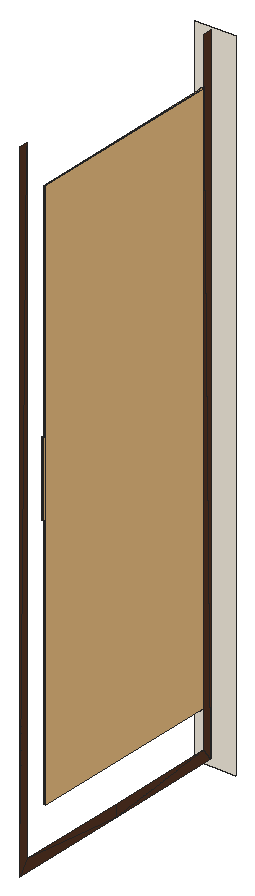
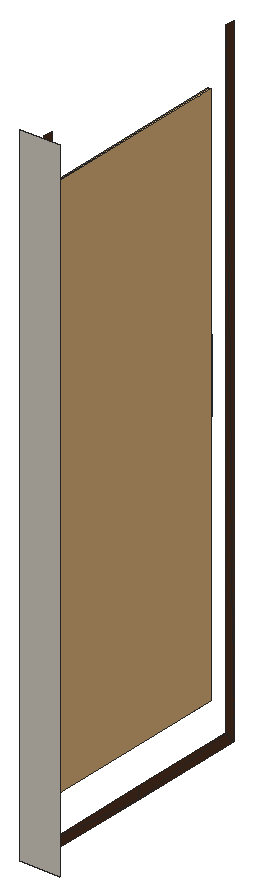
# SketchUp Ruby script. Lengths in inches.
U = 1.inch
M = Sketchup.active_model
def pt(a) = Geom::Point3d.new(a.map { |v| v * U })
def face(e, loops, mat)
  f = e.add_face(loops[0].map { |a| pt(a) })
  loops[1..].each { |l| e.add_face(l.map { |a| pt(a) }).erase! }
  f.material = f.back_material = mat if mat
  f
end
# faces: each face lists its corners as indices into pts; further lists are holes
def faces(e, pts, list, mat = nil) = list.each { |f| face(e, (f[0].is_a?(Array) ? f : [f]).map { |l| l.map { |i| pts[i] } }, mat) }
# xy, xz, yz: faces in a plane at the given z, y or x. An outline is a flat list of corners, or four numbers for a rectangle; further outlines are holes
def ring(l) = l.size == 4 ? [[l[0], l[1]], [l[2], l[1]], [l[2], l[3]], [l[0], l[3]]] : l.each_slice(2).to_a
def flat(e, list, mat, &to3) = list.each { |f| face(e, (f[0].is_a?(Array) ? f : [f]).map { |l| ring(l).map { |u, v| to3.(u, v) } }, mat) }
def xy(e, z, list, mat = nil) = flat(e, list, mat) { |x, y| [x, y, z] }
def xz(e, y, list, mat = nil) = flat(e, list, mat) { |x, z| [x, y, z] }
def yz(e, x, list, mat = nil) = flat(e, list, mat) { |y, z| [x, y, z] }
def lines(e, pts, list) = list.each { |a, b| e.add_line(pt(pts[a]), pt(pts[b])) }
# prism: a flat outline (further loops are holes) pulled along v
def prism(e, loops, v, mat = nil)
  f = face(e, loops, mat); d = Geom::Vector3d.new(v.map { |x| x * U })
  f.pushpull(f.normal.samedirection?(d) ? d.length : -d.length)
end
def box(e, o, s, mat = nil) = prism(e, [[o, [o[0] + s[0], o[1], o[2]], [o[0] + s[0], o[1] + s[1], o[2]], [o[0], o[1] + s[1], o[2]]]], [0, 0, s[2]], mat)
def at(x, y, z, deg = 0) = Geom::Transformation.translation(pt([x, y, z])) * Geom::Transformation.rotation(ORIGIN, Z_AXIS, deg.degrees)
def axes(o, x, y, z) = Geom::Transformation.new([*x, 0, *y, 0, *z, 0, *pt(o).to_a, 1])
def part(name) = M.definitions.add(name)
# library, detail: a bought-in or finely detailed component or shape, given as its bounding box
def library(name, o, s) = part(name).tap { |d| box(d.entities, o, s) }
def detail(e, o, s) = box(e.add_group.entities, o, s)
def put(e, d, t, mat = nil) = e.add_instance(d, t).tap { |i| i.material = mat if mat }
def group(e, t, mat = nil) = e.add_group.tap { |g| g.transformation = t; g.material = mat if mat }.entities
root = M.entities
M.materials.add("Material \#0").color = [86, 53, 35]
M.materials.add("Material \#1").color = [140, 140, 140]
M.materials.add("[0030_OldLace]").color = [253, 245, 230]
c1 = library("3DGeom~3_Defintion",[-83.33,-500,-350],[620.1,1000,533.33])
c2 = library("3DGeom~6_Defintion",[-5.59,-471.8,-48.03],[468.87,1000,73.72])
c3 = part("3DGeom~21_Defintion")
xy(c3.entities,73.08,[[-976.3,-241.71,23.7,-241.71,-976.3,-223.46],[23.7,-241.71,5.45,-223.46,-976.3,-223.46],[23.7,-241.71,23.7,0,5.45,-223.46],[5.45,-223.46,23.7,0,5.45,0],[23.7,0,23.7,241.71,5.45,223.46],
  [5.45,0,23.7,0,5.45,223.46],[-976.3,223.46,23.7,241.71,-976.3,241.71],[-976.3,223.46,5.45,223.46,23.7,241.71]],"Material \#0")
c4 = part("3DGeom~8_Defintion")
xz(c4.entities,-471.94,[[458.125,-17.29,459.53,-16.11,457.73,-17.15],[458.125,-17.29,458.54,-17.29,459.53,-16.11],[458.54,-17.29,458.93,-17.15,459.53,-16.11],[457.73,-17.15,459.53,-16.11,457.42,-16.88],[458.93,-17.15,459.25,-16.88,459.53,-16.11],
  [457.42,-16.88,459.53,-16.11,457.21,-16.52],[459.25,-16.88,459.46,-16.52,459.53,-16.11],[457.21,-16.52,459.53,-16.11,457.14,-16.11],[457.14,-16.11,459.53,-16.11,457.21,-15.7],[459.53,-16.11,457.42,-15.34,457.21,-15.7],
  [459.53,-16.11,457.73,-15.07,457.42,-15.34],[459.53,-16.11,458.125,-14.93,457.73,-15.07],[459.53,-16.11,458.54,-14.93,458.125,-14.93],[459.53,-16.11,458.93,-15.07,458.54,-14.93],[459.53,-16.11,459.25,-15.34,458.93,-15.07],
  [459.53,-16.11,459.46,-15.7,459.25,-15.34]],"Material \#1")
xz(c4.entities,-416.39,[[458.125,-17.29,457.73,-17.15,459.53,-16.11],[458.125,-17.29,459.53,-16.11,458.54,-17.29],[458.54,-17.29,459.53,-16.11,458.93,-17.15],[457.73,-17.15,457.42,-16.88,459.53,-16.11],[458.93,-17.15,459.53,-16.11,459.25,-16.88],
  [457.42,-16.88,457.21,-16.52,459.53,-16.11],[459.25,-16.88,459.53,-16.11,459.46,-16.52],[457.21,-16.52,457.14,-16.11,459.53,-16.11],[457.14,-16.11,457.21,-15.7,459.53,-16.11],[459.53,-16.11,457.21,-15.7,457.42,-15.34],
  [459.53,-16.11,457.42,-15.34,457.73,-15.07],[459.53,-16.11,457.73,-15.07,458.125,-14.93],[459.53,-16.11,458.125,-14.93,458.54,-14.93],[459.53,-16.11,458.54,-14.93,458.93,-15.07],[459.53,-16.11,458.93,-15.07,459.25,-15.34],
  [459.53,-16.11,459.25,-15.34,459.46,-15.7]],"Material \#1")
xz(c4.entities,-27.5,[[458.125,-17.29,459.53,-16.11,457.73,-17.15],[458.125,-17.29,458.54,-17.29,459.53,-16.11],[458.54,-17.29,458.93,-17.15,459.53,-16.11],[457.73,-17.15,459.53,-16.11,457.42,-16.88],[458.93,-17.15,459.25,-16.88,459.53,-16.11],
  [457.42,-16.88,459.53,-16.11,457.21,-16.52],[459.25,-16.88,459.46,-16.52,459.53,-16.11],[457.21,-16.52,459.53,-16.11,457.14,-16.11],[457.14,-16.11,459.53,-16.11,457.21,-15.7],[459.53,-16.11,457.42,-15.34,457.21,-15.7],
  [459.53,-16.11,457.73,-15.07,457.42,-15.34],[459.53,-16.11,458.125,-14.93,457.73,-15.07],[459.53,-16.11,458.54,-14.93,458.125,-14.93],[459.53,-16.11,458.93,-15.07,458.54,-14.93],[459.53,-16.11,459.25,-15.34,458.93,-15.07],
  [459.53,-16.11,459.46,-15.7,459.25,-15.34]],"Material \#1")
xz(c4.entities,28.06,[[458.125,-17.29,457.73,-17.15,459.53,-16.11],[458.125,-17.29,459.53,-16.11,458.54,-17.29],[458.54,-17.29,459.53,-16.11,458.93,-17.15],[457.73,-17.15,457.42,-16.88,459.53,-16.11],[458.93,-17.15,459.53,-16.11,459.25,-16.88],
  [457.42,-16.88,457.21,-16.52,459.53,-16.11],[459.25,-16.88,459.53,-16.11,459.46,-16.52],[457.21,-16.52,457.14,-16.11,459.53,-16.11],[457.14,-16.11,457.21,-15.7,459.53,-16.11],[459.53,-16.11,457.21,-15.7,457.42,-15.34],
  [459.53,-16.11,457.42,-15.34,457.73,-15.07],[459.53,-16.11,457.73,-15.07,458.125,-14.93],[459.53,-16.11,458.125,-14.93,458.54,-14.93],[459.53,-16.11,458.54,-14.93,458.93,-15.07],[459.53,-16.11,458.93,-15.07,459.25,-15.34],
  [459.53,-16.11,459.25,-15.34,459.46,-15.7]],"Material \#1")
xz(c4.entities,472.5,[[458.125,-17.29,459.53,-16.11,457.73,-17.15],[458.125,-17.29,458.54,-17.29,459.53,-16.11],[458.54,-17.29,458.93,-17.15,459.53,-16.11],[457.73,-17.15,459.53,-16.11,457.42,-16.88],[458.93,-17.15,459.25,-16.88,459.53,-16.11],
  [457.42,-16.88,459.53,-16.11,457.21,-16.52],[459.25,-16.88,459.46,-16.52,459.53,-16.11],[457.21,-16.52,459.53,-16.11,457.14,-16.11],[457.14,-16.11,459.53,-16.11,457.21,-15.7],[459.53,-16.11,457.42,-15.34,457.21,-15.7],
  [459.53,-16.11,457.73,-15.07,457.42,-15.34],[459.53,-16.11,458.125,-14.93,457.73,-15.07],[459.53,-16.11,458.54,-14.93,458.125,-14.93],[459.53,-16.11,458.93,-15.07,458.54,-14.93],[459.53,-16.11,459.25,-15.34,458.93,-15.07],
  [459.53,-16.11,459.46,-15.7,459.25,-15.34]],"Material \#1")
xz(c4.entities,528.06,[[458.125,-17.29,457.73,-17.15,459.53,-16.11],[458.125,-17.29,459.53,-16.11,458.54,-17.29],[458.54,-17.29,459.53,-16.11,458.93,-17.15],[457.73,-17.15,457.42,-16.88,459.53,-16.11],[458.93,-17.15,459.53,-16.11,459.25,-16.88],
  [457.42,-16.88,457.21,-16.52,459.53,-16.11],[459.25,-16.88,459.53,-16.11,459.46,-16.52],[457.21,-16.52,457.14,-16.11,459.53,-16.11],[457.14,-16.11,457.21,-15.7,459.53,-16.11],[459.53,-16.11,457.21,-15.7,457.42,-15.34],
  [459.53,-16.11,457.42,-15.34,457.73,-15.07],[459.53,-16.11,457.73,-15.07,458.125,-14.93],[459.53,-16.11,458.125,-14.93,458.54,-14.93],[459.53,-16.11,458.54,-14.93,458.93,-15.07],[459.53,-16.11,458.93,-15.07,459.25,-15.34],
  [459.53,-16.11,459.25,-15.34,459.46,-15.7]],"Material \#1")
c5 = library("3DGeom~9_Defintion",[456.52,-471.89,-18.89],[5.57,1000,5.49])
c6 = library("3DGeom~7_Defintion",[455.56,-471.94,-18.85],[5.55,1000,5.48])
xy(root,9.56,[[264.049,358.92,264.046,358.949,264.045,358.932],[264.049,358.92,264.049,358.939,264.046,358.949],[264.049,358.92,264.054,358.932,264.049,358.939],[264.045,358.932,264.042,358.978,264.041,358.964],[264.045,358.932,264.046,358.949,264.042,358.978],
  [264.054,358.932,264.053,358.949,264.049,358.939],[264.054,358.932,264.058,358.964,264.053,358.949],[264.053,358.949,264.058,358.964,264.057,358.978],[264.041,358.964,264.039,359.023,264.038,359.014],[264.041,358.964,264.042,358.978,264.039,359.023],
  [264.058,358.964,264.061,359.014,264.057,358.978],[264.057,358.978,264.061,359.014,264.059,359.023],[264.038,359.014,264.038,359.078,264.037,359.075],[264.038,359.014,264.039,359.023,264.038,359.078],[264.061,359.014,264.062,359.075,264.059,359.023],
  [264.059,359.023,264.062,359.075,264.061,359.078],[264.037,359.075,264.038,359.078,264.038,359.137],[264.037,359.075,264.038,359.137,264.037,359.14],[264.062,359.075,264.062,359.14,264.061,359.078],[264.061,359.078,264.062,359.14,264.061,359.137],
  [264.038,359.137,264.039,359.192,264.037,359.14],[264.061,359.137,264.061,359.201,264.059,359.192],[264.061,359.137,264.062,359.14,264.061,359.201],[264.037,359.14,264.039,359.192,264.038,359.201],[264.039,359.192,264.042,359.237,264.038,359.201],
  [264.059,359.192,264.058,359.251,264.057,359.237],[264.059,359.192,264.061,359.201,264.058,359.251],[264.038,359.201,264.042,359.237,264.041,359.251],[264.042,359.237,264.046,359.266,264.041,359.251],[264.057,359.237,264.054,359.284,264.053,359.266],
  [264.057,359.237,264.058,359.251,264.054,359.284],[264.041,359.251,264.046,359.266,264.045,359.284],[264.046,359.266,264.049,359.276,264.045,359.284],[264.053,359.266,264.049,359.295,264.049,359.276],[264.053,359.266,264.054,359.284,264.049,359.295],
  [264.049,359.276,264.049,359.295,264.045,359.284]],"Material \#1")
xy(root,9.58,[[264.049,358.92,264.045,358.932,264.049,358.939],[264.049,358.92,264.049,358.939,264.053,358.949],[264.049,358.92,264.053,358.949,264.054,358.932],[264.045,358.932,264.041,358.964,264.046,358.949],[264.045,358.932,264.046,358.949,264.049,358.939],
  [264.054,358.932,264.053,358.949,264.057,358.978],[264.054,358.932,264.057,358.978,264.058,358.964],[264.046,358.949,264.041,358.964,264.042,358.978],[264.041,358.964,264.038,359.014,264.042,358.978],[264.058,358.964,264.057,358.978,264.059,359.023],
  [264.058,358.964,264.059,359.023,264.061,359.014],[264.042,358.978,264.038,359.014,264.039,359.023],[264.038,359.014,264.037,359.075,264.039,359.023],[264.061,359.014,264.059,359.023,264.061,359.078],[264.061,359.014,264.061,359.078,264.062,359.075],
  [264.039,359.023,264.037,359.075,264.038,359.078],[264.037,359.075,264.037,359.14,264.038,359.078],[264.062,359.075,264.061,359.078,264.061,359.137],[264.062,359.075,264.061,359.137,264.062,359.14],[264.038,359.078,264.037,359.14,264.038,359.137],
  [264.038,359.137,264.037,359.14,264.038,359.201],[264.038,359.137,264.038,359.201,264.039,359.192],[264.061,359.137,264.059,359.192,264.062,359.14],[264.062,359.14,264.059,359.192,264.061,359.201],[264.039,359.192,264.038,359.201,264.041,359.251],
  [264.039,359.192,264.041,359.251,264.042,359.237],[264.059,359.192,264.057,359.237,264.061,359.201],[264.061,359.201,264.057,359.237,264.058,359.251],[264.042,359.237,264.041,359.251,264.045,359.284],[264.042,359.237,264.045,359.284,264.046,359.266],
  [264.057,359.237,264.053,359.266,264.058,359.251],[264.058,359.251,264.053,359.266,264.054,359.284],[264.046,359.266,264.045,359.284,264.049,359.295],[264.046,359.266,264.049,359.295,264.049,359.276],[264.053,359.266,264.049,359.276,264.054,359.284],
  [264.049,359.276,264.049,359.295,264.054,359.284]],"Material \#1")
xy(root,14.023,[[264.049,358.92,264.049,358.939,264.045,358.932],[264.049,358.92,264.053,358.949,264.049,358.939],[264.049,358.92,264.054,358.932,264.053,358.949],[264.045,358.932,264.046,358.949,264.041,358.964],[264.045,358.932,264.049,358.939,264.046,358.949],
  [264.054,358.932,264.057,358.978,264.053,358.949],[264.054,358.932,264.058,358.964,264.057,358.978],[264.046,358.949,264.042,358.978,264.041,358.964],[264.041,358.964,264.042,358.978,264.038,359.014],[264.058,358.964,264.059,359.023,264.057,358.978],
  [264.058,358.964,264.061,359.014,264.059,359.023],[264.042,358.978,264.039,359.023,264.038,359.014],[264.038,359.014,264.039,359.023,264.037,359.075],[264.061,359.014,264.061,359.078,264.059,359.023],[264.061,359.014,264.062,359.075,264.061,359.078],
  [264.039,359.023,264.038,359.078,264.037,359.075],[264.037,359.075,264.038,359.078,264.037,359.14],[264.062,359.075,264.061,359.137,264.061,359.078],[264.062,359.075,264.062,359.14,264.061,359.137],[264.038,359.078,264.038,359.137,264.037,359.14],
  [264.038,359.137,264.038,359.201,264.037,359.14],[264.038,359.137,264.039,359.192,264.038,359.201],[264.061,359.137,264.062,359.14,264.059,359.192],[264.062,359.14,264.061,359.201,264.059,359.192],[264.039,359.192,264.041,359.251,264.038,359.201],
  [264.039,359.192,264.042,359.237,264.041,359.251],[264.059,359.192,264.061,359.201,264.057,359.237],[264.061,359.201,264.058,359.251,264.057,359.237],[264.042,359.237,264.045,359.284,264.041,359.251],[264.042,359.237,264.046,359.266,264.045,359.284],
  [264.057,359.237,264.058,359.251,264.053,359.266],[264.058,359.251,264.054,359.284,264.053,359.266],[264.046,359.266,264.049,359.295,264.045,359.284],[264.046,359.266,264.049,359.276,264.049,359.295],[264.053,359.266,264.054,359.284,264.049,359.276],
  [264.049,359.276,264.054,359.284,264.049,359.295]],"Material \#1")
xy(root,14.043,[[264.049,358.92,264.045,358.932,264.046,358.949],[264.049,358.92,264.046,358.949,264.049,358.939],[264.049,358.92,264.049,358.939,264.054,358.932],[264.045,358.932,264.041,358.964,264.042,358.978],[264.045,358.932,264.042,358.978,264.046,358.949],
  [264.054,358.932,264.049,358.939,264.053,358.949],[264.054,358.932,264.053,358.949,264.058,358.964],[264.053,358.949,264.057,358.978,264.058,358.964],[264.041,358.964,264.038,359.014,264.039,359.023],[264.041,358.964,264.039,359.023,264.042,358.978],
  [264.058,358.964,264.057,358.978,264.061,359.014],[264.057,358.978,264.059,359.023,264.061,359.014],[264.038,359.014,264.037,359.075,264.038,359.078],[264.038,359.014,264.038,359.078,264.039,359.023],[264.061,359.014,264.059,359.023,264.062,359.075],
  [264.059,359.023,264.061,359.078,264.062,359.075],[264.037,359.075,264.037,359.14,264.038,359.137],[264.037,359.075,264.038,359.137,264.038,359.078],[264.062,359.075,264.061,359.078,264.062,359.14],[264.061,359.078,264.061,359.137,264.062,359.14],
  [264.038,359.137,264.037,359.14,264.039,359.192],[264.061,359.137,264.059,359.192,264.061,359.201],[264.061,359.137,264.061,359.201,264.062,359.14],[264.037,359.14,264.038,359.201,264.039,359.192],[264.039,359.192,264.038,359.201,264.042,359.237],
  [264.059,359.192,264.057,359.237,264.058,359.251],[264.059,359.192,264.058,359.251,264.061,359.201],[264.038,359.201,264.041,359.251,264.042,359.237],[264.042,359.237,264.041,359.251,264.046,359.266],[264.057,359.237,264.053,359.266,264.054,359.284],
  [264.057,359.237,264.054,359.284,264.058,359.251],[264.041,359.251,264.045,359.284,264.046,359.266],[264.046,359.266,264.045,359.284,264.049,359.276],[264.053,359.266,264.049,359.276,264.049,359.295],[264.053,359.266,264.049,359.295,264.054,359.284],
  [264.049,359.276,264.045,359.284,264.049,359.295]],"Material \#1")
xy(root,54.139,[[264.049,358.92,264.046,358.949,264.045,358.932],[264.049,358.92,264.049,358.939,264.046,358.949],[264.049,358.92,264.054,358.932,264.049,358.939],[264.045,358.932,264.042,358.978,264.041,358.964],[264.045,358.932,264.046,358.949,264.042,358.978],
  [264.054,358.932,264.053,358.949,264.049,358.939],[264.054,358.932,264.058,358.964,264.053,358.949],[264.053,358.949,264.058,358.964,264.057,358.978],[264.041,358.964,264.039,359.023,264.038,359.014],[264.041,358.964,264.042,358.978,264.039,359.023],
  [264.058,358.964,264.061,359.014,264.057,358.978],[264.057,358.978,264.061,359.014,264.059,359.023],[264.038,359.014,264.038,359.078,264.037,359.075],[264.038,359.014,264.039,359.023,264.038,359.078],[264.061,359.014,264.062,359.075,264.059,359.023],
  [264.059,359.023,264.062,359.075,264.061,359.078],[264.037,359.075,264.038,359.078,264.038,359.137],[264.037,359.075,264.038,359.137,264.037,359.14],[264.062,359.075,264.062,359.14,264.061,359.078],[264.061,359.078,264.062,359.14,264.061,359.137],
  [264.038,359.137,264.039,359.192,264.037,359.14],[264.061,359.137,264.061,359.201,264.059,359.192],[264.061,359.137,264.062,359.14,264.061,359.201],[264.037,359.14,264.039,359.192,264.038,359.201],[264.039,359.192,264.042,359.237,264.038,359.201],
  [264.059,359.192,264.058,359.251,264.057,359.237],[264.059,359.192,264.061,359.201,264.058,359.251],[264.038,359.201,264.042,359.237,264.041,359.251],[264.042,359.237,264.046,359.266,264.041,359.251],[264.057,359.237,264.054,359.284,264.053,359.266],
  [264.057,359.237,264.058,359.251,264.054,359.284],[264.041,359.251,264.046,359.266,264.045,359.284],[264.046,359.266,264.049,359.276,264.045,359.284],[264.053,359.266,264.049,359.295,264.049,359.276],[264.053,359.266,264.054,359.284,264.049,359.295],
  [264.049,359.276,264.049,359.295,264.045,359.284]],"Material \#1")
xy(root,54.159,[[264.049,358.92,264.045,358.932,264.049,358.939],[264.049,358.92,264.049,358.939,264.053,358.949],[264.049,358.92,264.053,358.949,264.054,358.932],[264.045,358.932,264.041,358.964,264.046,358.949],[264.045,358.932,264.046,358.949,264.049,358.939],
  [264.054,358.932,264.053,358.949,264.057,358.978],[264.054,358.932,264.057,358.978,264.058,358.964],[264.046,358.949,264.041,358.964,264.042,358.978],[264.041,358.964,264.038,359.014,264.042,358.978],[264.058,358.964,264.057,358.978,264.059,359.023],
  [264.058,358.964,264.059,359.023,264.061,359.014],[264.042,358.978,264.038,359.014,264.039,359.023],[264.038,359.014,264.037,359.075,264.039,359.023],[264.061,359.014,264.059,359.023,264.061,359.078],[264.061,359.014,264.061,359.078,264.062,359.075],
  [264.039,359.023,264.037,359.075,264.038,359.078],[264.037,359.075,264.037,359.14,264.038,359.078],[264.062,359.075,264.061,359.078,264.061,359.137],[264.062,359.075,264.061,359.137,264.062,359.14],[264.038,359.078,264.037,359.14,264.038,359.137],
  [264.038,359.137,264.037,359.14,264.038,359.201],[264.038,359.137,264.038,359.201,264.039,359.192],[264.061,359.137,264.059,359.192,264.062,359.14],[264.062,359.14,264.059,359.192,264.061,359.201],[264.039,359.192,264.038,359.201,264.041,359.251],
  [264.039,359.192,264.041,359.251,264.042,359.237],[264.059,359.192,264.057,359.237,264.061,359.201],[264.061,359.201,264.057,359.237,264.058,359.251],[264.042,359.237,264.041,359.251,264.045,359.284],[264.042,359.237,264.045,359.284,264.046,359.266],
  [264.057,359.237,264.053,359.266,264.058,359.251],[264.058,359.251,264.053,359.266,264.054,359.284],[264.046,359.266,264.045,359.284,264.049,359.295],[264.046,359.266,264.049,359.295,264.049,359.276],[264.053,359.266,264.049,359.276,264.054,359.284],
  [264.049,359.276,264.049,359.295,264.054,359.284]],"Material \#1")
xz(root,361.777,[[261,0,267.4375,106]],"[0030_OldLace]")
yz(root,263.952,[[328.295,50.6,328.293,50.614,328.406,50.64],[328.293,50.614,328.402,50.654,328.406,50.64],[328.406,50.64,328.402,50.654,328.508,50.704],[328.402,50.654,328.502,50.717,328.508,50.704],[328.508,50.704,328.502,50.717,328.6,50.79],
  [328.502,50.717,328.592,50.801,328.6,50.79],[328.6,50.79,328.592,50.801,328.679,50.894],[328.592,50.801,328.67,50.904,328.679,50.894],[328.679,50.894,328.67,50.904,328.743,51.015],[328.67,50.904,328.734,51.023,328.743,51.015],
  [328.335,50.93,328.355,50.968,328.365,50.96],[328.365,50.96,328.355,50.968,328.381,51.005],[328.355,50.968,328.371,51.01,328.381,51.005],[328.381,51.005,328.371,51.01,328.392,51.054],[328.371,51.01,328.38,51.057,328.392,51.054],
  [328.743,51.015,328.734,51.023,328.792,51.15],[328.734,51.023,328.781,51.155,328.792,51.15],[328.392,51.054,328.38,51.057,328.395,51.105],[328.38,51.057,328.384,51.105,328.395,51.105],[328.384,51.105,328.38,51.154,328.392,51.157],
  [328.384,51.105,328.392,51.157,328.395,51.105],[328.792,51.15,328.781,51.155,328.822,51.296],[328.38,51.154,328.371,51.201,328.381,51.206],[328.38,51.154,328.381,51.206,328.392,51.157],[328.781,51.155,328.811,51.299,328.822,51.296],
  [328.371,51.201,328.355,51.243,328.365,51.251],[328.371,51.201,328.365,51.251,328.381,51.206],[328.822,51.296,328.811,51.299,328.833,51.458],[328.811,51.299,328.822,51.458,328.833,51.458]],"Material \#1")
yz(root,264.101,[[328.177,50.586,328.295,50.6,328.177,50.601],[328.295,50.6,328.293,50.614,328.177,50.601],[328.295,50.6,328.406,50.64,328.293,50.614],[328.293,50.614,328.406,50.64,328.402,50.654],[328.406,50.64,328.508,50.704,328.402,50.654],
  [328.402,50.654,328.508,50.704,328.502,50.717],[328.508,50.704,328.6,50.79,328.502,50.717],[328.502,50.717,328.6,50.79,328.592,50.801],[328.6,50.79,328.679,50.894,328.592,50.801],[328.592,50.801,328.679,50.894,328.67,50.904],
  [328.216,50.822,328.214,50.837,328.177,50.832],[328.216,50.822,328.253,50.836,328.214,50.837],[328.253,50.836,328.249,50.85,328.214,50.837],[328.253,50.836,328.287,50.857,328.249,50.85],[328.249,50.85,328.287,50.857,328.281,50.87],
  [328.287,50.857,328.318,50.885,328.281,50.87],[328.281,50.87,328.318,50.885,328.31,50.897],[328.318,50.885,328.344,50.92,328.31,50.897],[328.679,50.894,328.743,51.015,328.67,50.904],[328.31,50.897,328.344,50.92,328.335,50.93],
  [328.67,50.904,328.743,51.015,328.734,51.023],[328.344,50.92,328.365,50.96,328.335,50.93],[328.335,50.93,328.365,50.96,328.355,50.968],[328.365,50.96,328.381,51.005,328.355,50.968],[328.355,50.968,328.381,51.005,328.371,51.01],
  [328.381,51.005,328.392,51.054,328.371,51.01],[328.371,51.01,328.392,51.054,328.38,51.057],[328.743,51.015,328.792,51.15,328.734,51.023],[328.734,51.023,328.792,51.15,328.781,51.155],[328.392,51.054,328.395,51.105,328.38,51.057],
  [328.38,51.057,328.395,51.105,328.384,51.105],[328.384,51.105,328.392,51.157,328.38,51.154],[328.384,51.105,328.395,51.105,328.392,51.157],[328.792,51.15,328.822,51.296,328.781,51.155],[328.38,51.154,328.381,51.206,328.371,51.201],
  [328.38,51.154,328.392,51.157,328.381,51.206],[328.781,51.155,328.822,51.296,328.811,51.299],[328.371,51.201,328.365,51.251,328.355,51.243],[328.371,51.201,328.381,51.206,328.365,51.251],[328.355,51.243,328.344,51.291,328.335,51.281],
  [328.355,51.243,328.365,51.251,328.344,51.291],[328.335,51.281,328.318,51.325,328.31,51.314],[328.335,51.281,328.344,51.291,328.318,51.325],[328.822,51.296,328.833,51.458,328.811,51.299],[328.811,51.299,328.833,51.458,328.822,51.458],
  [328.31,51.314,328.287,51.354,328.281,51.341],[328.31,51.314,328.318,51.325,328.287,51.354],[328.281,51.341,328.253,51.375,328.249,51.361],[328.281,51.341,328.287,51.354,328.253,51.375],[328.249,51.361,328.216,51.389,328.214,51.374],
  [328.249,51.361,328.253,51.375,328.216,51.389],[328.214,51.374,328.216,51.389,328.177,51.393],[328.822,51.458,328.833,51.458,328.833,61.353],[328.822,51.458,328.833,61.353,328.822,53.591],[328.822,53.591,328.833,61.353,328.822,61.352]],"Material \#1")
put(root,c1,axes([263.98,328.18,56.41],[0,0.009,0],[0,0,-0.01189],[-0.00061,0,0]),"Material \#1")
put(root,c2,axes([263.98,328.18,56.41],[0,0.06713,0],[0,0,-0.08869],[-0.00458,0,0]),"Material \#1")
put(root,c3,axes([263.65,342.05,3.9],[0,0,-0.10451],[0,0.07911,0],[0.0054,0,0]),"Material \#0")
put(root,c4,axes([263.98,328.18,56.41],[0,0.06748,0],[0,0,-0.08916],[-0.00461,0,0]),"Material \#1")
put(root,c5,axes([263.98,328.18,56.41],[0,0.06734,0],[0,0,-0.08897],[-0.0046,0,0]),"Material \#1")
put(root,c6,axes([263.98,328.18,56.41],[0,0.06748,0],[0,0,-0.08916],[-0.00461,0,0]),"Material \#1")
